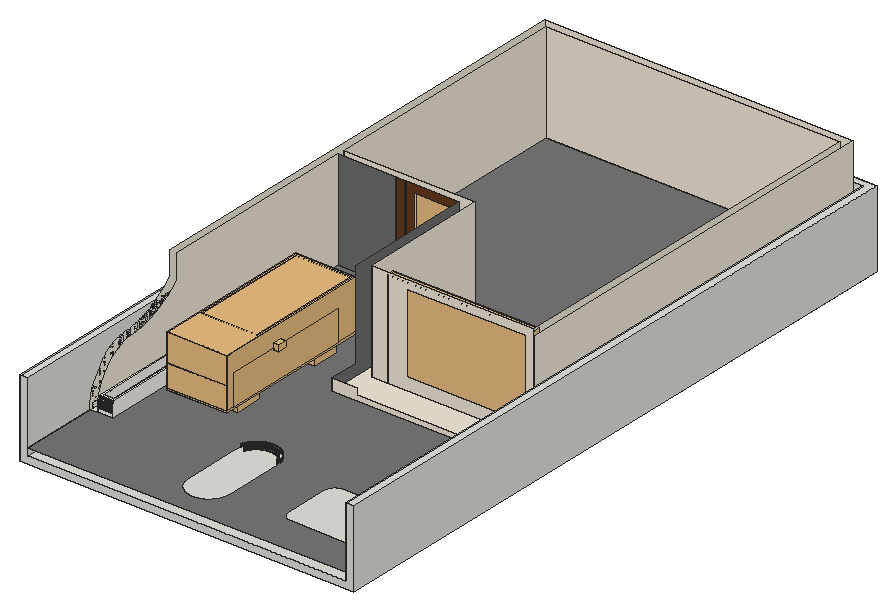
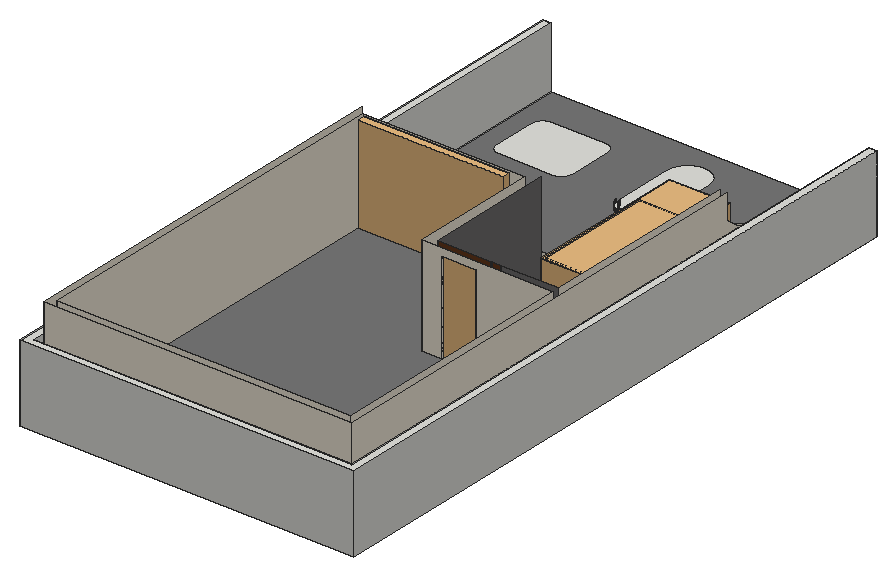
# SketchUp Ruby script. Lengths in inches.
U = 1.inch
M = Sketchup.active_model
def pt(a) = Geom::Point3d.new(a.map { |v| v * U })
def face(e, loops, mat)
  f = e.add_face(loops[0].map { |a| pt(a) })
  loops[1..].each { |l| e.add_face(l.map { |a| pt(a) }).erase! }
  f.material = f.back_material = mat if mat
  f
end
# faces: each face lists its corners as indices into pts; further lists are holes
def faces(e, pts, list, mat = nil) = list.each { |f| face(e, (f[0].is_a?(Array) ? f : [f]).map { |l| l.map { |i| pts[i] } }, mat) }
# xy, xz, yz: faces in a plane at the given z, y or x. An outline is a flat list of corners, or four numbers for a rectangle; further outlines are holes
def ring(l) = l.size == 4 ? [[l[0], l[1]], [l[2], l[1]], [l[2], l[3]], [l[0], l[3]]] : l.each_slice(2).to_a
def flat(e, list, mat, &to3) = list.each { |f| face(e, (f[0].is_a?(Array) ? f : [f]).map { |l| ring(l).map { |u, v| to3.(u, v) } }, mat) }
def xy(e, z, list, mat = nil) = flat(e, list, mat) { |x, y| [x, y, z] }
def xz(e, y, list, mat = nil) = flat(e, list, mat) { |x, z| [x, y, z] }
def yz(e, x, list, mat = nil) = flat(e, list, mat) { |y, z| [x, y, z] }
def lines(e, pts, list) = list.each { |a, b| e.add_line(pt(pts[a]), pt(pts[b])) }
# prism: a flat outline (further loops are holes) pulled along v
def prism(e, loops, v, mat = nil)
  f = face(e, loops, mat); d = Geom::Vector3d.new(v.map { |x| x * U })
  f.pushpull(f.normal.samedirection?(d) ? d.length : -d.length)
end
def box(e, o, s, mat = nil) = prism(e, [[o, [o[0] + s[0], o[1], o[2]], [o[0] + s[0], o[1] + s[1], o[2]], [o[0], o[1] + s[1], o[2]]]], [0, 0, s[2]], mat)
def at(x, y, z, deg = 0) = Geom::Transformation.translation(pt([x, y, z])) * Geom::Transformation.rotation(ORIGIN, Z_AXIS, deg.degrees)
def axes(o, x, y, z) = Geom::Transformation.new([*x, 0, *y, 0, *z, 0, *pt(o).to_a, 1])
def part(name) = M.definitions.add(name)
# library, detail: a bought-in or finely detailed component or shape, given as its bounding box
def library(name, o, s) = part(name).tap { |d| box(d.entities, o, s) }
def detail(e, o, s) = box(e.add_group.entities, o, s)
def put(e, d, t, mat = nil) = e.add_instance(d, t).tap { |i| i.material = mat if mat }
def group(e, t, mat = nil) = e.add_group.tap { |g| g.transformation = t; g.material = mat if mat }.entities
root = M.entities
M.materials.add("0027 AP L140 CRUSHED ICE").color = [241, 233, 217]
M.materials.add("Black_matte").color = [7, 7, 7]
M.materials.add("False ceiling Light").color = [253, 207, 127]
M.materials.add("Glass_headlight").color = [127, 127, 127]
M.materials["Glass_headlight"].alpha = 0.29
M.materials.add("[Metal Seamed]").color = [40, 40, 40]
M.materials.add("[Quartz Light Grey]").color = [248, 243, 236]
M.materials.add("[Slate Light Tile]").color = [119, 119, 119]
M.materials.add("[Stone Vein Gray]").color = [112, 111, 111]
M.materials.add("[Wood Cherry Original]").color = [103, 58, 28]
c1 = library("Wheel1",[-0.22,0.28,-1.22],[12.14,34.32,34.67])
c2 = library("Group\#47",[0,0,0],[81,26.91,31.48])
c3 = library("Group\#46",[0,-11.74,0],[75.48,151.34,31.8125])
c4 = library("Group\#45",[0,0,0],[59.24,11.61,17.61])
c5 = library("Group\#48",[0,0,0],[83.57,167.11,42.22])
c6 = library("Group\#49",[0,0,0],[97.91,11.39,8.3])
c7 = library("Group\#50",[0,0,0],[82.49,206.98,67.77])
c8 = library("Group\#51",[0,0,0],[82.02,206.91,71.71])
c9 = part("l405 Vogue 2013")
put(c9.entities,c1,axes([23.09,177.11,0.71],[-1.08,0,0],[0,-1,0],[0,0,1]))
put(c9.entities,c1,axes([83.66,53.48,1.89],[1.08,0,0],[0,-1,0],[0,0,1]))
put(c9.entities,c1,axes([23.09,53.48,1.89],[-1.08,0,0],[0,-1,0],[0,0,1]))
put(c9.entities,c1,axes([83.66,177.11,0.71],[1.08,0,0],[0,-1,0],[0,0,1]))
put(c9.entities,c2,axes([97.16,27.0625,11.6],[-1.08,0,0],[0,-1,0],[0,0,1]))
put(c9.entities,c3,axes([94.18,192.03,48.94],[-1.08,0,0],[0,-1,0],[0,0,1]),"Glass_headlight")
put(c9.entities,c4,axes([85.41,206.68,30.35],[-1.08,0,0],[0,-1,0],[0,0,1]))
put(c9.entities,c5,axes([98.55,177.66,12.76],[-1.08,0,0],[0,-1,0],[0,0,1]))
put(c9.entities,c6,axes([106.29,85.5,53.72],[-1.08,0,0],[0,-1,0],[0,0,1]))
put(c9.entities,c7,axes([97.96,207.84,12.8],[-1.08,0,0],[0,-1,0],[0,0,1]))
put(c9.entities,c8,axes([97.7,207.32,9.05],[-1.08,0,0],[0,-1,0],[0,0,1]))
c10 = part("2013 Land Rover Range Rover l405")
put(c10.entities,c9,axes([0,0,0],[1,0,0],[0,1.03,0],[0,0,1]),"Black_matte")
c11 = part("2014+Range+Rover+l405+UK-version+ISA")
put(c11.entities,c10,at(0,0,0),"Black_matte")
c12 = library("Curtains",[0,0,0],[121.73,8.19,117.22])
c13 = library("Group\#3",[0,-2.5,0],[42,5.95,111])
xy(root,-9,[[9,0,393,780]])
xy(root,0,[[9,94,18,214],[9,214,9,780,381,780,381,264,165,264,165,456,153,456,153,465,177,465,177,309,372,309,372,771,18,771,18,465,111,465,111,456,100,456,100,456.5,99,456.5,99,456,88,456,88,456.5,18,456.5,18,214]],"0027 AP L140 CRUSHED ICE")
xy(root,0,[[[9,0,393,780],[291,44,290.59,44.01,290.18,44.03,289.78,44.06,289.37,44.1,288.97,44.16,288.5625,44.23,288.16,44.3125,287.77,44.41,287.375,44.52,286.98,44.64,286.6,44.77,286.21,44.91,285.84,45.07,285.46,45.24,285.1,45.42,284.74,45.61,284.38,45.81,284.03,46.02,283.69,46.25,283.36,46.48,283.03,46.73,282.71,46.98,282.4,47.25,282.1,47.52,281.52,48.1,281.25,48.4,280.98,48.71,280.73,49.03,280.48,49.36,280.25,49.69,280.02,50.03,279.81,50.38,279.61,50.74,279.42,51.1,279.24,51.46,279.07,51.84,278.91,52.21,278.77,52.6,278.64,52.98,278.52,53.375,278.41,53.77,278.3125,54.16,278.23,54.5625,278.16,54.97,278.1,55.37,278.06,55.78,278.03,56.18,278.01,56.59,278,57,278,111,278.01,111.41,278.03,111.82,278.06,112.22,278.1,112.63,278.16,113.03,278.23,113.4375,278.3125,113.84,278.41,114.23,278.52,114.625,278.64,115.02,278.77,115.4,278.91,115.79,279.07,116.16,279.24,116.54,279.42,116.9,279.61,117.26,279.81,117.62,280.02,117.97,280.25,118.31,280.48,118.64,280.73,118.97,280.98,119.29,281.25,119.6,281.52,119.9,282.1,120.48,282.4,120.75,282.71,121.02,283.03,121.27,283.36,121.52,283.69,121.75,284.03,121.98,284.38,122.19,284.74,122.39,285.1,122.58,285.46,122.76,285.84,122.93,286.21,123.09,286.6,123.23,286.98,123.36,287.375,123.48,287.77,123.59,288.16,123.6875,288.5625,123.77,288.97,123.84,289.37,123.9,289.78,123.94,290.18,123.97,290.59,123.99,291,124,357,124,357.41,123.99,357.82,123.97,358.22,123.94,358.63,123.9,359.03,123.84,359.4375,123.77,359.84,123.6875,360.23,123.59,360.625,123.48,361.02,123.36,361.4,123.23,361.79,123.09,362.16,122.93,362.54,122.76,362.9,122.58,363.26,122.39,363.62,122.19,363.97,121.98,364.31,121.75,364.64,121.52,364.97,121.27,365.29,121.02,365.6,120.75,365.9,120.48,366.48,119.9,366.75,119.6,367.02,119.29,367.27,118.97,367.52,118.64,367.75,118.31,367.98,117.97,368.19,117.62,368.39,117.26,368.58,116.9,368.76,116.54,368.93,116.16,369.09,115.79,369.23,115.4,369.36,115.02,369.48,114.625,369.59,114.23,369.6875,113.84,369.77,113.4375,369.84,113.03,369.9,112.63,369.94,112.22,369.97,111.82,369.99,111.41,370,111,370,57,369.99,56.59,369.97,56.18,369.94,55.78,369.9,55.37,369.84,54.97,369.77,54.5625,369.6875,54.16,369.59,53.77,369.48,53.375,369.36,52.98,369.23,52.6,369.09,52.21,368.93,51.84,368.76,51.46,368.58,51.1,368.39,50.74,368.19,50.38,367.98,50.03,367.75,49.69,367.52,49.36,367.27,49.03,367.02,48.71,366.75,48.4,366.48,48.1,365.9,47.52,365.6,47.25,365.29,46.98,364.97,46.73,364.64,46.48,364.31,46.25,363.97,46.02,363.62,45.81,363.26,45.61,362.9,45.42,362.54,45.24,362.16,45.07,361.79,44.91,361.4,44.77,361.02,44.64,360.625,44.52,360.23,44.41,359.84,44.3125,359.4375,44.23,359.03,44.16,358.63,44.1,358.22,44.06,357.82,44.03,357.41,44.01,357,44],[189,23,188.35,23.01,187.69,23.03,187.04,23.08,186.39,23.14,185.74,23.21,185.09,23.31,184.44,23.42,183.8,23.55,183.16,23.69,182.53,23.85,181.9,24.03,181.27,24.22,180.65,24.43,180.04,24.66,179.43,24.9,178.83,25.16,177.65,25.72,177.07,26.03,176.5,26.35,175.9375,26.68,175.38,27.03,174.84,27.4,174.31,27.77,173.78,28.17,173.27,28.57,172.76,28.99,172.27,29.42,171.79,29.87,171.32,30.32,170.87,30.79,170.42,31.27,169.99,31.76,169.57,32.27,169.17,32.78,168.77,33.31,168.4,33.84,168.03,34.38,167.68,34.9375,167.35,35.5,167.03,36.07,166.72,36.65,166.16,37.83,165.9,38.43,165.66,39.04,165.43,39.65,165.22,40.27,165.03,40.9,164.85,41.53,164.69,42.16,164.55,42.8,164.42,43.44,164.31,44.09,164.21,44.74,164.14,45.39,164.08,46.04,164.03,46.69,164.01,47.35,164,48,164,120,164.01,120.65,164.03,121.31,164.08,121.96,164.14,122.61,164.21,123.26,164.31,123.91,164.42,124.56,164.55,125.2,164.69,125.84,164.85,126.47,165.03,127.1,165.22,127.73,165.43,128.35,165.66,128.96,165.9,129.57,166.16,130.17,166.72,131.35,167.03,131.93,167.35,132.5,167.68,133.0625,168.03,133.62,168.4,134.16,168.77,134.69,169.17,135.22,169.57,135.73,169.99,136.24,170.42,136.73,170.87,137.21,171.32,137.68,171.79,138.13,172.27,138.58,172.76,139.01,173.27,139.43,173.78,139.83,174.31,140.23,174.84,140.6,175.38,140.97,175.9375,141.32,176.5,141.65,177.07,141.97,177.65,142.28,178.83,142.84,179.43,143.1,180.04,143.34,180.65,143.57,181.27,143.78,181.9,143.97,182.53,144.15,183.16,144.31,183.8,144.45,184.44,144.58,185.09,144.69,185.74,144.79,186.39,144.86,187.04,144.92,187.69,144.97,188.35,144.99,189,145,189.65,144.99,190.31,144.97,190.96,144.92,191.61,144.86,192.26,144.79,192.91,144.69,193.56,144.58,194.2,144.45,194.84,144.31,195.47,144.15,196.1,143.97,196.73,143.78,197.35,143.57,197.96,143.34,198.57,143.1,199.17,142.84,200.35,142.28,200.93,141.97,201.5,141.65,202.0625,141.32,202.62,140.97,203.16,140.6,203.69,140.23,204.22,139.83,204.73,139.43,205.24,139.01,205.73,138.58,206.21,138.13,206.68,137.68,207.13,137.21,207.58,136.73,208.01,136.24,208.43,135.73,208.83,135.22,209.23,134.69,209.6,134.16,209.97,133.62,210.32,133.0625,210.65,132.5,210.97,131.93,211.28,131.35,211.84,130.17,212.1,129.57,212.34,128.96,212.57,128.35,212.78,127.73,212.97,127.1,213.15,126.47,213.31,125.84,213.45,125.2,213.58,124.56,213.69,123.91,213.79,123.26,213.86,122.61,213.92,121.96,213.97,121.31,213.99,120.65,214,120,214,48,213.99,47.35,213.97,46.69,213.92,46.04,213.86,45.39,213.79,44.74,213.69,44.09,213.58,43.44,213.45,42.8,213.31,42.16,213.15,41.53,212.97,40.9,212.78,40.27,212.57,39.65,212.34,39.04,212.1,38.43,211.84,37.83,211.28,36.65,210.97,36.07,210.65,35.5,210.32,34.9375,209.97,34.38,209.6,33.84,209.23,33.31,208.83,32.78,208.43,32.27,208.01,31.76,207.58,31.27,207.13,30.79,206.68,30.32,206.21,29.87,205.73,29.42,205.24,28.99,204.73,28.57,204.22,28.17,203.69,27.77,203.16,27.4,202.62,27.03,202.0625,26.68,201.5,26.35,200.93,26.03,200.35,25.72,199.17,25.16,198.57,24.9,197.96,24.66,197.35,24.43,196.73,24.22,196.1,24.03,195.47,23.85,194.84,23.69,194.2,23.55,193.56,23.42,192.91,23.31,192.26,23.21,191.61,23.14,190.96,23.08,190.31,23.03,189.65,23.01]]],"[Slate Light Tile]")
xz(root,264,[[165,0,381,0,381,14,354,14,354,6,195,6,195,14,165,14]],"0027 AP L140 CRUSHED ICE")
xz(root,309,[[[177,0,372,120],[219,14,363,110]]],"0027 AP L140 CRUSHED ICE")
xz(root,456,[[88,0,99,120],[100,0,111,0,111,111,153,111,153,0,165,0,165,120,100,120]],"[Wood Cherry Original]")
xz(root,456.5,[[99,0,100,120]],"0027 AP L140 CRUSHED ICE")
xz(root,456.5,[[18,0,88,120]],"[Stone Vein Gray]")
xz(root,465,[[18,0,18,120,177,120,177,0,153,0,153,111,111,111,111,0]],"0027 AP L140 CRUSHED ICE")
xz(root,771,[[18,0,372,120]],"0027 AP L140 CRUSHED ICE")
xz(root,780,[[9,-9,393,0]])
xz(root,780,[[9,0,381,120]],"0027 AP L140 CRUSHED ICE")
yz(root,9,[[0,-9,780,0]])
yz(root,9,[[94,0,94,4.5,94.01,4.73,94.04,5.41,94.08,6.08,94.13,6.76,94.18,7.43,94.24,8.1,94.31,8.78,94.39,9.45,94.57,10.79,94.67,11.46,94.78,12.125,94.9,12.79,95.02,13.45,95.15,14.12,95.43,15.44,95.75,16.76,95.92,17.41,96.09,18.0625,96.28,18.71,96.66,20.01,96.87,20.65,97.08,21.3,97.3,21.93,97.76,23.21,98.01,23.84,98.25,24.47,98.77,25.71,99.04,26.33,99.6,27.57,99.89,28.18,100.19,28.78,100.5,29.39,100.81,29.99,101.125,30.58,101.45,31.18,101.78,31.76,102.12,32.35,102.82,33.51,103.54,34.65,103.91,35.22,104.29,35.78,104.67,36.33,105.0625,36.89,105.46,37.43,105.86,37.98,106.27,38.52,106.6875,39.05,107.11,39.58,107.53,40.1,107.97,40.625,108.41,41.14,108.85,41.65,109.3,42.15,109.76,42.65,110.22,43.14,111.16,44.12,111.64,44.6,112.12,45.07,112.61,45.53,113.1,46,113.6,46.45,114.62,47.35,115.13,47.79,115.65,48.22,116.17,48.64,116.7,49.07,117.78,49.89,118.32,50.29,118.87,50.6875,119.42,51.08,120.54,51.84,121.1,52.21,121.67,52.57,122.25,52.93,122.82,53.28,123.4,53.63,123.99,53.97,124.58,54.3,125.17,54.625,125.77,54.94,126.97,55.56,127.58,55.86,128.19,56.15,128.8,56.43,129.42,56.71,130.04,56.98,131.46,57.56,132.9,58.08,134.35,58.55,135.83,58.98,137.3125,59.34,138.8125,59.65,140.32,59.91,141.15,60.02,141.84,60.12,143.36,60.27,144.89,60.36,146.42,60.4,147.95,60.38,148.64,60.4375,149.33,60.5,150.01,60.57,150.7,60.64,151.38,60.72,152.07,60.8,152.75,60.89,153.4375,60.98,154.12,61.07,155.48,61.27,156.17,61.38,156.85,61.49,158.21,61.73,158.88,61.85,159.5625,61.98,160.24,62.11,160.91,62.25,161.59,62.39,162.26,62.54,162.94,62.6875,163.61,62.84,164.95,63.16,166.29,63.5,166.95,63.68,167.62,63.86,168.28,64.04,168.95,64.23,169.61,64.42,171.59,65.02,172.24,65.23,172.9,65.44,173.55,65.66,174.21,65.88,176.16,66.57,176.81,66.81,177.45,67.05,178.1,67.3,179.38,67.8,180.66,68.32,181.29,68.59,181.93,68.86,182.56,69.13,183.82,69.69,184.45,69.98,185.07,70.27,185.7,70.5625,186.32,70.86,186.9375,71.16,187.56,71.47,188.17,71.78,188.79,72.09,190.01,72.73,190.62,73.06,191.22,73.38,191.83,73.72,192.43,74.05,193.03,74.39,194.22,75.09,194.8125,75.4375,195.41,75.79,195.99,76.15,196.58,76.52,197.16,76.88,197.75,77.25,198.32,77.63,199.48,78.39,200.05,78.77,201.19,79.55,201.75,79.95,202.3125,80.35,202.87,80.75,203.43,81.16,203.98,81.57,204.54,81.98,205.08,82.4,206.18,83.24,207.26,84.1,207.79,84.53,208.85,85.41,209.38,85.86,209.91,86.3,210.43,86.75,210.95,87.21,211.46,87.67,211.98,88.125,212.49,88.59,212.99,89.06,213.5,89.53,214,90,214,120,780,120,780,0]],"0027 AP L140 CRUSHED ICE")
yz(root,18,[[94,0,456.5,0,456.5,120,214,120,214,90,213.5,89.53,212.99,89.06,212.49,88.59,211.98,88.125,211.46,87.67,210.95,87.21,210.43,86.75,209.91,86.3,209.38,85.86,208.85,85.41,207.79,84.53,207.26,84.1,206.18,83.24,205.08,82.4,204.54,81.98,203.98,81.57,203.43,81.16,202.87,80.75,202.3125,80.35,201.75,79.95,201.19,79.55,200.05,78.77,199.48,78.39,198.32,77.63,197.75,77.25,197.16,76.88,196.58,76.52,195.99,76.15,195.41,75.79,194.8125,75.4375,194.22,75.09,193.03,74.39,192.43,74.05,191.83,73.72,191.22,73.38,190.62,73.06,190.01,72.73,188.79,72.09,188.17,71.78,187.56,71.47,186.9375,71.16,186.32,70.86,185.7,70.5625,185.07,70.27,184.45,69.98,183.82,69.69,182.56,69.13,181.93,68.86,181.29,68.59,180.66,68.32,179.38,67.8,178.1,67.3,177.45,67.05,176.81,66.81,176.16,66.57,174.21,65.88,173.55,65.66,172.9,65.44,172.24,65.23,171.59,65.02,169.61,64.42,168.95,64.23,168.28,64.04,167.62,63.86,166.95,63.68,166.29,63.5,164.95,63.16,163.61,62.84,162.94,62.6875,162.26,62.54,161.59,62.39,160.91,62.25,160.24,62.11,159.5625,61.98,158.88,61.85,158.21,61.73,156.85,61.49,156.17,61.38,155.48,61.27,154.12,61.07,153.4375,60.98,152.75,60.89,152.07,60.8,151.38,60.72,150.7,60.64,150.01,60.57,149.33,60.5,148.64,60.4375,147.95,60.38,146.42,60.4,144.89,60.36,143.36,60.27,141.84,60.12,141.15,60.02,140.32,59.91,138.8125,59.65,137.3125,59.34,135.83,58.98,134.35,58.55,132.9,58.08,131.46,57.56,130.04,56.98,129.42,56.71,128.8,56.43,128.19,56.15,127.58,55.86,126.97,55.56,125.77,54.94,125.17,54.625,124.58,54.3,123.99,53.97,123.4,53.63,122.82,53.28,122.25,52.93,121.67,52.57,121.1,52.21,120.54,51.84,119.42,51.08,118.87,50.6875,118.32,50.29,117.78,49.89,116.7,49.07,116.17,48.64,115.65,48.22,115.13,47.79,114.62,47.35,113.6,46.45,113.1,46,112.61,45.53,112.12,45.07,111.64,44.6,111.16,44.12,110.22,43.14,109.76,42.65,109.3,42.15,108.85,41.65,108.41,41.14,107.97,40.625,107.53,40.1,107.11,39.58,106.6875,39.05,106.27,38.52,105.86,37.98,105.46,37.43,105.0625,36.89,104.67,36.33,104.29,35.78,103.91,35.22,103.54,34.65,102.82,33.51,102.12,32.35,101.78,31.76,101.45,31.18,101.125,30.58,100.81,29.99,100.5,29.39,100.19,28.78,99.89,28.18,99.6,27.57,99.04,26.33,98.77,25.71,98.25,24.47,98.01,23.84,97.76,23.21,97.3,21.93,97.08,21.3,96.87,20.65,96.66,20.01,96.28,18.71,96.09,18.0625,96.08,18,95.92,17.41,95.75,16.76,95.43,15.44,95.15,14.12,95.02,13.45,94.9,12.79,94.78,12.125,94.67,11.46,94.57,10.79,94.39,9.45,94.31,8.78,94.24,8.1,94.18,7.43,94.13,6.76,94.08,6.08,94.04,5.41,94.01,4.73,94,4.5],[465,0,771,120]],"0027 AP L140 CRUSHED ICE")
yz(root,88,[[456,0,456.5,120]],"0027 AP L140 CRUSHED ICE")
yz(root,99,[[456,0,456.5,120]],"0027 AP L140 CRUSHED ICE")
yz(root,100,[[456,0,456.5,120]],"0027 AP L140 CRUSHED ICE")
yz(root,111,[[456,0,465,111]],"0027 AP L140 CRUSHED ICE")
yz(root,153,[[456,0,465,111]],"0027 AP L140 CRUSHED ICE")
yz(root,165,[[264,0,264,14,300,14,300,120,456,120,456,0]],"[Stone Vein Gray]")
yz(root,177,[[309,0,465,120]],"0027 AP L140 CRUSHED ICE")
yz(root,372,[[309,0,771,120]],"0027 AP L140 CRUSHED ICE")
yz(root,381,[[264,0,780,0,780,120,300,120,300,14,264,14]],"0027 AP L140 CRUSHED ICE")
yz(root,393,[[0,-9,780,0]])
p = [[169.03,126.49,-3],[169.03,126.49,3],[168.86,125.96,3],[168.86,125.96,-3],[209.14,125.96,-3],[209.14,125.96,3],
  [208.97,126.49,3],[208.97,126.49,-3],[169.2,127.01,-3],[169.2,127.01,3],[208.8,127.01,3],[208.8,127.01,-3],
  [169.39,127.53,-3],[169.39,127.53,3],[208.61,127.53,3],[208.61,127.53,-3],[169.6,128.04,-3],[169.6,128.04,3],
  [208.4,128.04,3],[208.4,128.04,-3],[169.82,128.54,-3],[169.82,128.54,3],[208.18,128.54,3],[208.18,128.54,-3],
  [170.05,129.04,-3],[170.05,129.04,3],[207.95,129.04,3],[207.95,129.04,-3],[170.29,129.53,-3],[170.29,129.53,3],
  [207.71,129.53,3],[207.71,129.53,-3],[170.54,130.02,-3],[170.54,130.02,3],[207.46,130.02,3],[207.46,130.02,-3],
  [170.8125,130.5,-3],[170.8125,130.5,3],[207.1875,130.5,3],[207.1875,130.5,-3],[171.09,130.97,-3],[171.09,130.97,3],
  [206.91,130.97,3],[206.91,130.97,-3],[171.39,131.4375,-3],[171.39,131.4375,3],[206.61,131.4375,3],[206.61,131.4375,-3],
  [171.69,131.89,-3],[171.69,131.89,3],[206.31,131.89,3],[206.31,131.89,-3],[172.01,132.34,-3],[172.01,132.34,3],
  [205.99,132.34,3],[205.99,132.34,-3],[172.34,132.78,-3],[172.34,132.78,3],[205.66,132.78,3],[205.66,132.78,-3],
  [172.68,133.22,-3],[172.68,133.22,3],[205.32,133.22,3],[205.32,133.22,-3],[173.03,133.64,-3],[173.03,133.64,3],
  [204.97,133.64,3],[204.97,133.64,-3],[173.39,134.05,-3],[173.39,134.05,3],[204.61,134.05,3],[204.61,134.05,-3],
  [173.77,134.46,-3],[173.77,134.46,3],[204.23,134.46,3],[204.23,134.46,-3],[174.15,134.85,-3],[174.15,134.85,3],
  [203.85,134.85,3],[203.85,134.85,-3],[174.54,135.23,-3],[174.54,135.23,3],[203.46,135.23,3],[203.46,135.23,-3],
  [174.95,135.61,-3],[174.95,135.61,3],[203.05,135.61,3],[203.05,135.61,-3],[175.36,135.97,-3],[175.36,135.97,3],
  [202.64,135.97,3],[202.64,135.97,-3],[175.78,136.32,-3],[175.78,136.32,3],[202.22,136.32,3],[202.22,136.32,-3],
  [176.22,136.66,-3],[176.22,136.66,3],[201.78,136.66,3],[201.78,136.66,-3],[176.66,136.99,-3],[176.66,136.99,3],
  [201.34,136.99,3],[201.34,136.99,-3],[177.11,137.31,-3],[177.11,137.31,3],[200.89,137.31,3],[200.89,137.31,-3],
  [177.5625,137.61,-3],[177.5625,137.61,3],[200.4375,137.61,3],[200.4375,137.61,-3],[178.03,137.91,-3],[178.03,137.91,3],
  [199.97,137.91,3],[199.97,137.91,-3],[178.5,138.1875,-3],[178.5,138.1875,3],[199.5,138.1875,3],[199.5,138.1875,-3],
  [178.98,138.46,-3],[178.98,138.46,3],[199.02,138.46,3],[199.02,138.46,-3],[179.47,138.71,-3],[179.47,138.71,3],
  [198.53,138.71,3],[198.53,138.71,-3],[179.96,138.95,-3],[179.96,138.95,3],[198.04,138.95,3],[198.04,138.95,-3],
  [180.46,139.18,-3],[180.46,139.18,3],[197.54,139.18,3],[197.54,139.18,-3],[180.96,139.4,-3],[180.96,139.4,3],
  [197.04,139.4,3],[197.04,139.4,-3],[181.47,139.61,-3],[181.47,139.61,3],[196.53,139.61,3],[196.53,139.61,-3],
  [181.99,139.8,-3],[181.99,139.8,3],[196.01,139.8,3],[196.01,139.8,-3],[182.51,139.97,-3],[182.51,139.97,3],
  [195.49,139.97,3],[195.49,139.97,-3],[183.04,140.14,-3],[183.04,140.14,3],[194.96,140.14,3],[194.96,140.14,-3],
  [183.56,140.28,-3],[183.56,140.28,3],[194.44,140.28,3],[194.44,140.28,-3],[184.1,140.42,-3],[184.1,140.42,3],
  [193.9,140.42,3],[193.9,140.42,-3],[184.63,140.54,-3],[184.63,140.54,3],[193.37,140.54,3],[193.37,140.54,-3],
  [185.17,140.65,-3],[185.17,140.65,3],[192.83,140.65,3],[192.83,140.65,-3],[185.71,140.74,-3],[185.71,140.74,3],
  [192.29,140.74,3],[192.29,140.74,-3],[186.26,140.82,-3],[186.26,140.82,3],[191.74,140.82,3],[191.74,140.82,-3],
  [186.8,140.88,-3],[186.8,140.88,3],[191.2,140.88,3],[191.2,140.88,-3],[187.35,140.94,-3],[187.35,140.94,3],
  [187.9,140.97,-3],[187.9,140.97,3],[190.65,140.94,-3],[190.65,140.94,3],[190.1,140.97,3],[190.1,140.97,-3],
  [188.45,140.99,-3],[188.45,140.99,3],[189,141,-3],[189,141,3],[189.55,140.99,-3],[189.55,140.99,3],
  [213.31,125.84,0],[213.15,126.47,0],[213.15,126.47,3],[213.31,125.84,3],[165.03,127.1,0],[164.85,126.47,0],
  [164.85,126.47,3],[165.03,127.1,3],[212.97,127.1,0],[212.97,127.1,3],[165.22,127.73,0],[165.22,127.73,3],
  [212.78,127.73,0],[212.78,127.73,3],[165.43,128.35,0],[165.43,128.35,3],[212.57,128.35,0],[212.57,128.35,3],
  [165.66,128.96,0],[165.66,128.96,3],[212.34,128.96,0],[212.34,128.96,3],[165.9,129.57,0],[165.9,129.57,3],
  [212.1,129.57,0],[212.1,129.57,3],[166.16,130.17,0],[166.16,130.17,3],[211.84,130.17,0],[211.84,130.17,3],
  [166.44,130.76,0],[166.44,130.76,3],[211.56,130.76,0],[211.56,130.76,3],[166.72,131.35,0],[166.72,131.35,3],
  [211.28,131.35,0],[211.28,131.35,3],[167.03,131.93,0],[167.03,131.93,3],[210.97,131.93,0],[210.97,131.93,3],
  [167.35,132.5,0],[167.35,132.5,3],[210.65,132.5,0],[210.65,132.5,3],[167.68,133.0625,0],[167.68,133.0625,3],
  [210.32,133.0625,0],[210.32,133.0625,3],[168.03,133.62,0],[168.03,133.62,3],[209.97,133.62,0],[209.97,133.62,3],
  [168.4,134.16,0],[168.4,134.16,3],[209.6,134.16,0],[209.6,134.16,3],[168.77,134.69,0],[168.77,134.69,3],
  [209.23,134.69,0],[209.23,134.69,3],[169.17,135.22,0],[169.17,135.22,3],[208.83,135.22,0],[208.83,135.22,3],
  [169.57,135.73,0],[169.57,135.73,3],[208.43,135.73,0],[208.43,135.73,3],[169.99,136.24,0],[169.99,136.24,3],
  [208.01,136.24,0],[208.01,136.24,3],[170.42,136.73,0],[170.42,136.73,3],[207.58,136.73,0],[207.58,136.73,3],
  [170.87,137.21,0],[170.87,137.21,3],[207.13,137.21,0],[207.13,137.21,3],[171.32,137.68,0],[171.32,137.68,3],
  [206.68,137.68,0],[206.68,137.68,3],[171.79,138.13,0],[171.79,138.13,3],[206.21,138.13,0],[206.21,138.13,3],
  [172.27,138.58,0],[172.27,138.58,3],[205.73,138.58,0],[205.73,138.58,3],[172.76,139.01,0],[172.76,139.01,3],
  [205.24,139.01,0],[205.24,139.01,3],[173.27,139.43,0],[173.27,139.43,3],[204.73,139.43,0],[204.73,139.43,3],
  [173.78,139.83,0],[173.78,139.83,3],[204.22,139.83,0],[204.22,139.83,3],[174.31,140.23,0],[174.31,140.23,3],
  [203.69,140.23,0],[203.69,140.23,3],[174.84,140.6,0],[174.84,140.6,3],[203.16,140.6,0],[203.16,140.6,3],
  [175.38,140.97,0],[175.38,140.97,3],[202.62,140.97,0],[202.62,140.97,3],[175.9375,141.32,0],[175.9375,141.32,3],
  [202.0625,141.32,0],[202.0625,141.32,3],[176.5,141.65,0],[176.5,141.65,3],[201.5,141.65,0],[201.5,141.65,3],
  [177.07,141.97,0],[177.07,141.97,3],[200.93,141.97,0],[200.93,141.97,3],[177.65,142.28,0],[177.65,142.28,3],
  [200.35,142.28,0],[200.35,142.28,3],[178.24,142.56,0],[178.24,142.56,3],[199.76,142.56,0],[199.76,142.56,3],
  [178.83,142.84,0],[178.83,142.84,3],[199.17,142.84,0],[199.17,142.84,3],[179.43,143.1,0],[179.43,143.1,3],
  [198.57,143.1,0],[198.57,143.1,3],[180.04,143.34,0],[180.04,143.34,3],[197.96,143.34,0],[197.96,143.34,3],
  [180.65,143.57,0],[180.65,143.57,3],[197.35,143.57,0],[197.35,143.57,3],[181.27,143.78,0],[181.27,143.78,3],
  [196.73,143.78,0],[196.73,143.78,3],[181.9,143.97,0],[181.9,143.97,3],[196.1,143.97,0],[196.1,143.97,3],
  [182.53,144.15,0],[182.53,144.15,3],[195.47,144.15,0],[195.47,144.15,3],[183.16,144.31,0],[183.16,144.31,3],
  [194.84,144.31,0],[194.84,144.31,3],[183.8,144.45,0],[183.8,144.45,3],[194.2,144.45,0],[194.2,144.45,3],
  [184.44,144.58,0],[184.44,144.58,3],[193.56,144.58,0],[193.56,144.58,3],[185.09,144.69,0],[185.09,144.69,3],
  [192.91,144.69,0],[192.91,144.69,3],[185.74,144.79,0],[185.74,144.79,3],[192.26,144.79,0],[192.26,144.79,3],
  [186.39,144.86,0],[186.39,144.86,3],[191.61,144.86,0],[191.61,144.86,3],[187.04,144.92,0],[187.04,144.92,3],
  [187.69,144.97,0],[187.69,144.97,3],[190.96,144.92,0],[190.31,144.97,0],[190.31,144.97,3],[190.96,144.92,3],
  [188.35,144.99,0],[188.35,144.99,3],[189,145,0],[189,145,3],[189.65,144.99,0],[189.65,144.99,3]]
faces(root,p,[[0,1,2,3],[4,5,6,7],[8,9,1,0],[7,6,10,11],[12,13,9,8],[11,10,14,15],[16,17,13,12],[15,14,18,19],
  [20,21,17,16],[19,18,22,23],[24,25,21,20],[23,22,26,27],[28,29,25,24],[27,26,30,31],[32,33,29,28],[31,30,34,35],
  [36,37,33,32],[35,34,38,39],[40,41,37,36],[39,38,42,43],[44,45,41,40],[43,42,46,47],[48,49,45,44],[47,46,50,51],
  [52,53,49,48],[51,50,54,55],[56,57,53,52],[55,54,58,59],[60,61,57,56],[59,58,62,63],[64,65,61,60],[63,62,66,67],
  [68,69,65,64],[67,66,70,71],[72,73,69,68],[71,70,74,75],[76,77,73,72],[75,74,78,79],[80,81,77,76],[79,78,82,83],
  [84,85,81,80],[83,82,86,87],[88,89,85,84],[87,86,90,91],[92,93,89,88],[91,90,94,95],[96,97,93,92],[95,94,98,99],
  [100,101,97,96],[99,98,102,103],[104,105,101,100],[103,102,106,107],[108,109,105,104],[107,106,110,111],[112,113,109,108],[111,110,114,115],
  [116,117,113,112],[115,114,118,119],[120,121,117,116],[119,118,122,123],[124,125,121,120],[123,122,126,127],[128,129,125,124],[127,126,130,131],
  [132,133,129,128],[131,130,134,135],[136,137,133,132],[135,134,138,139],[140,141,137,136],[139,138,142,143],[144,145,141,140],[143,142,146,147],
  [148,149,145,144],[147,146,150,151],[152,153,149,148],[151,150,154,155],[156,157,153,152],[155,154,158,159],[160,161,157,156],[159,158,162,163],
  [164,165,161,160],[163,162,166,167],[168,169,165,164],[167,166,170,171],[172,173,169,168],[171,170,174,175],[176,177,173,172],[175,174,178,179],
  [180,181,177,176],[179,178,182,183],[184,185,181,180],[186,187,185,184],[188,189,190,191],[183,182,189,188],[192,193,187,186],[194,195,193,192],
  [196,197,195,194],[191,190,197,196],[198,199,200,201],[202,203,204,205],[199,206,207,200],[208,202,205,209],[206,210,211,207],[212,208,209,213],
  [210,214,215,211],[216,212,213,217],[214,218,219,215],[220,216,217,221],[218,222,223,219],[224,220,221,225],[222,226,227,223],[228,224,225,229],
  [226,230,231,227],[232,228,229,233],[230,234,235,231],[236,232,233,237],[234,238,239,235],[240,236,237,241],[238,242,243,239],[244,240,241,245],
  [242,246,247,243],[248,244,245,249],[246,250,251,247],[252,248,249,253],[250,254,255,251],[256,252,253,257],[254,258,259,255],[260,256,257,261],
  [258,262,263,259],[264,260,261,265],[262,266,267,263],[268,264,265,269],[266,270,271,267],[272,268,269,273],[270,274,275,271],[276,272,273,277],
  [274,278,279,275],[280,276,277,281],[278,282,283,279],[284,280,281,285],[282,286,287,283],[288,284,285,289],[286,290,291,287],[292,288,289,293],
  [290,294,295,291],[296,292,293,297],[294,298,299,295],[300,296,297,301],[298,302,303,299],[304,300,301,305],[302,306,307,303],[308,304,305,309],
  [306,310,311,307],[312,308,309,313],[310,314,315,311],[316,312,313,317],[314,318,319,315],[320,316,317,321],[318,322,323,319],[324,320,321,325],
  [322,326,327,323],[328,324,325,329],[326,330,331,327],[332,328,329,333],[330,334,335,331],[336,332,333,337],[334,338,339,335],[340,336,337,341],
  [338,342,343,339],[344,340,341,345],[342,346,347,343],[348,344,345,349],[346,350,351,347],[352,348,349,353],[350,354,355,351],[356,352,353,357],
  [354,358,359,355],[360,356,357,361],[358,362,363,359],[364,360,361,365],[362,366,367,363],[368,364,365,369],[366,370,371,367],[372,368,369,373],
  [370,374,375,371],[376,372,373,377],[374,378,379,375],[380,376,377,381],[378,382,383,379],[384,380,381,385],[382,386,387,383],[388,384,385,389],
  [390,388,389,391],[392,393,394,395],[386,392,395,387],[396,390,391,397],[398,396,397,399],[400,398,399,401],[393,400,401,394]],"[Slate Light Tile]")
g1 = group(root,at(18,94,0),"[Quartz Light Grey]")
xy(g1,0,[[0,0,18,110.5]])
xy(g1,2,[[3,5.08,15,107.5]])
xy(g1,18,[[[0,2.08,18,110.5],[3,5.08,15,107.5]]])
xz(g1,0,[[0,0,18,4.5]])
xz(g1,5.08,[[3,2,15,18]])
xz(g1,107.5,[[3,2,15,18]])
xz(g1,110.5,[[0,0,18,18]])
yz(g1,0,[[0,0,0,4.5,0.01,4.73,0.04,5.41,0.08,6.08,0.13,6.76,0.18,7.43,0.24,8.1,0.31,8.78,0.39,9.45,0.57,10.79,0.67,11.46,0.78,12.125,0.9,12.79,1.02,13.45,1.15,14.12,1.43,15.44,1.75,16.76,1.92,17.41,2.08,18,110.5,18,110.5,0]])
yz(g1,3,[[5.08,2,107.5,18]])
yz(g1,15,[[5.08,2,107.5,18]])
yz(g1,18,[[0,0,110.5,0,110.5,18,2.08,18,1.92,17.41,1.75,16.76,1.43,15.44,1.15,14.12,1.02,13.45,0.9,12.79,0.78,12.125,0.67,11.46,0.57,10.79,0.39,9.45,0.31,8.78,0.24,8.1,0.18,7.43,0.13,6.76,0.08,6.08,0.04,5.41,0.01,4.73,0,4.5]])
p = [[0,0.01,4.73],[0,0,4.5],[18,0,4.5],[18,0.01,4.73],[0,0.04,5.41],[18,0.04,5.41],
  [0,0.08,6.08],[18,0.08,6.08],[0,0.13,6.76],[18,0.13,6.76],[0,0.18,7.43],[18,0.18,7.43],
  [0,0.24,8.1],[18,0.24,8.1],[0,0.31,8.78],[18,0.31,8.78],[0,0.39,9.45],[18,0.39,9.45],
  [0,0.48,10.12],[18,0.48,10.12],[0,0.57,10.79],[18,0.57,10.79],[0,0.67,11.46],[18,0.67,11.46],
  [0,0.78,12.125],[18,0.78,12.125],[0,0.9,12.79],[18,0.9,12.79],[0,1.02,13.45],[18,1.02,13.45],
  [0,1.15,14.12],[18,1.15,14.12],[0,1.29,14.78],[18,1.29,14.78],[0,1.43,15.44],[18,1.43,15.44],
  [0,1.59,16.1],[18,1.59,16.1],[0,1.75,16.76],[18,1.75,16.76],[0,1.92,17.41],[18,1.92,17.41],
  [0,2.08,18],[18,2.08,18]]
faces(g1,p,[[0,1,2,3],[4,0,3,5],[6,4,5,7],[8,6,7,9],[10,8,9,11],[12,10,11,13],[14,12,13,15],[16,14,15,17],
  [18,16,17,19],[20,18,19,21],[22,20,21,23],[24,22,23,25],[26,24,25,27],[28,26,27,29],[30,28,29,31],[32,30,31,33],
  [34,32,33,35],[36,34,35,37],[38,36,37,39],[40,38,39,41],[42,40,41,43]])
put(root,c11,axes([42.78,158,-0.07],[0.8184,0,0],[0,0.91,0],[0,0,0.86765]))
put(root,c12,axes([196.43,309,0],[1.44235,0,0],[0,1,0],[0,0,1]),"0027 AP L140 CRUSHED ICE")
g2 = group(root,at(9,0,-9))
xy(g2,-9,[[-9,0,393,789]])
xy(g2,0,[[0,0,384,780]])
xy(g2,84,[[-9,0,0,0,0,780,384,780,384,0,393,0,393,789,-9,789]])
xz(g2,0,[[-9,-9,393,-9,393,84,384,84,384,0,0,0,0,84,-9,84]])
xz(g2,780,[[0,0,384,84]])
xz(g2,789,[[-9,-9,393,84]])
yz(g2,-9,[[0,-9,789,84]])
yz(g2,0,[[0,0,780,84]])
yz(g2,384,[[0,0,780,84]])
yz(g2,393,[[0,-9,789,84]])
g3 = group(root,at(99,456.5,0),"False ceiling Light")
box(g3,[0,-0.5,0],[1,0.5,120])
put(root,c13,at(111,460,0),"[Metal Seamed]")
